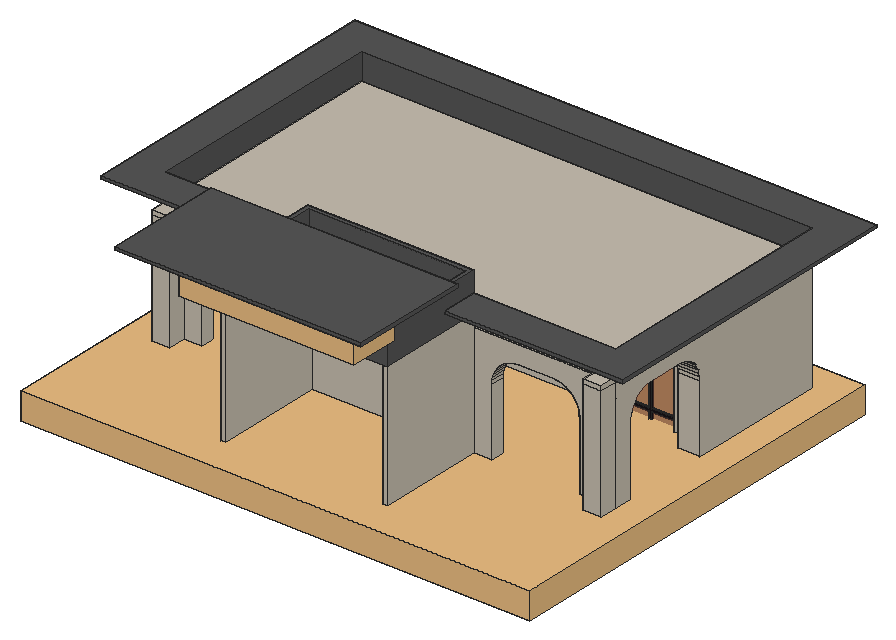
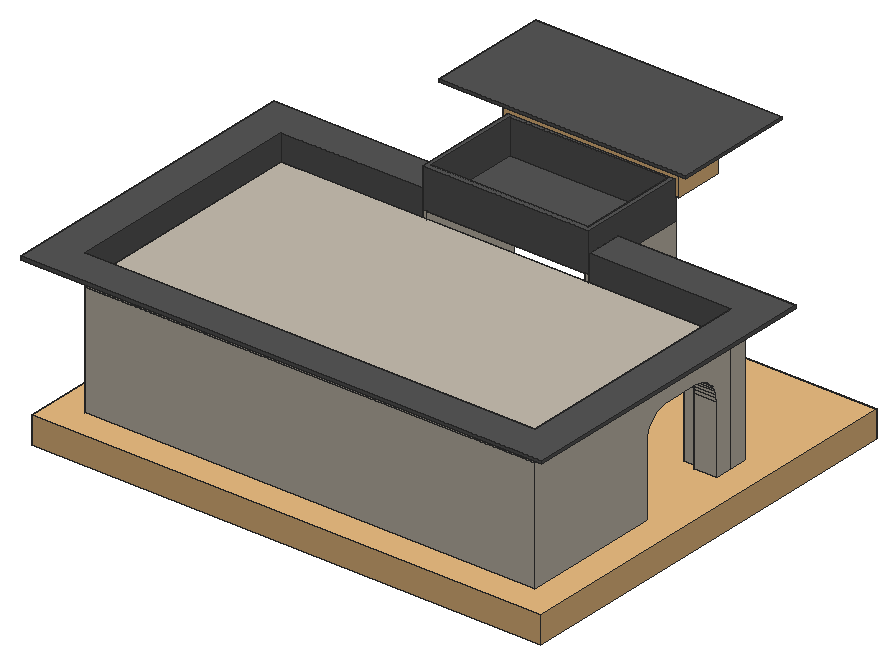
# SketchUp Ruby script. Lengths in inches.
U = 1.inch
M = Sketchup.active_model
def pt(a) = Geom::Point3d.new(a.map { |v| v * U })
def face(e, loops, mat)
  f = e.add_face(loops[0].map { |a| pt(a) })
  loops[1..].each { |l| e.add_face(l.map { |a| pt(a) }).erase! }
  f.material = f.back_material = mat if mat
  f
end
# faces: each face lists its corners as indices into pts; further lists are holes
def faces(e, pts, list, mat = nil) = list.each { |f| face(e, (f[0].is_a?(Array) ? f : [f]).map { |l| l.map { |i| pts[i] } }, mat) }
# xy, xz, yz: faces in a plane at the given z, y or x. An outline is a flat list of corners, or four numbers for a rectangle; further outlines are holes
def ring(l) = l.size == 4 ? [[l[0], l[1]], [l[2], l[1]], [l[2], l[3]], [l[0], l[3]]] : l.each_slice(2).to_a
def flat(e, list, mat, &to3) = list.each { |f| face(e, (f[0].is_a?(Array) ? f : [f]).map { |l| ring(l).map { |u, v| to3.(u, v) } }, mat) }
def xy(e, z, list, mat = nil) = flat(e, list, mat) { |x, y| [x, y, z] }
def xz(e, y, list, mat = nil) = flat(e, list, mat) { |x, z| [x, y, z] }
def yz(e, x, list, mat = nil) = flat(e, list, mat) { |y, z| [x, y, z] }
def lines(e, pts, list) = list.each { |a, b| e.add_line(pt(pts[a]), pt(pts[b])) }
# prism: a flat outline (further loops are holes) pulled along v
def prism(e, loops, v, mat = nil)
  f = face(e, loops, mat); d = Geom::Vector3d.new(v.map { |x| x * U })
  f.pushpull(f.normal.samedirection?(d) ? d.length : -d.length)
end
def box(e, o, s, mat = nil) = prism(e, [[o, [o[0] + s[0], o[1], o[2]], [o[0] + s[0], o[1] + s[1], o[2]], [o[0], o[1] + s[1], o[2]]]], [0, 0, s[2]], mat)
def at(x, y, z, deg = 0) = Geom::Transformation.translation(pt([x, y, z])) * Geom::Transformation.rotation(ORIGIN, Z_AXIS, deg.degrees)
def axes(o, x, y, z) = Geom::Transformation.new([*x, 0, *y, 0, *z, 0, *pt(o).to_a, 1])
def part(name) = M.definitions.add(name)
# library, detail: a bought-in or finely detailed component or shape, given as its bounding box
def library(name, o, s) = part(name).tap { |d| box(d.entities, o, s) }
def detail(e, o, s) = box(e.add_group.entities, o, s)
def put(e, d, t, mat = nil) = e.add_instance(d, t).tap { |i| i.material = mat if mat }
def group(e, t, mat = nil) = e.add_group.tap { |g| g.transformation = t; g.material = mat if mat }.entities
root = M.entities
M.materials.add("[0034_Wheat]").color = [198, 190, 175]
M.materials.add("[Carrera Marble]").color = [207, 207, 207]
M.materials.add("[Color M06]").color = [86, 86, 86]
M.materials.add("[Color M07]").color = [25, 20, 24]
M.materials.add("[Translucent Glass Dark Green]").color = [114, 59, 48]
M.materials["[Translucent Glass Dark Green]"].alpha = 0.5
c1 = library("Group\#14",[0,0,0],[679.6,559.6,36])
c2 = part("window")
xy(c2.entities,0,[[0,0,117,2]])
xy(c2.entities,3,[[3,0,38.5,2],[38.5,0,41.5,2],[41.5,0,75.5,2],[75.5,0,78.5,2],[78.5,0,114,2]])
xy(c2.entities,33,[[3,0,38.5,2],[41.5,0,75.5,2],[78.5,0,114,2]])
xy(c2.entities,36,[[3,0,38.5,2],[41.5,0,75.5,2],[78.5,0,114,2]])
xy(c2.entities,96,[[3,0,38.5,2],[41.5,0,75.5,2],[78.5,0,114,2]])
xy(c2.entities,99,[[3,0,38.5,2],[41.5,0,75.5,2],[78.5,0,114,2]])
xy(c2.entities,129,[[3,0,38.5,2],[41.5,0,75.5,2],[78.5,0,114,2]])
xy(c2.entities,132,[[0,0,117,2]])
xz(c2.entities,0,[[[0,0,117,132],[3,3,3,33,38.5,33,38.5,3,41.5,3,41.5,33,75.5,33,75.5,3,78.5,3,78.5,33,114,33,114,3],[3,36,38.5,96],[78.5,36,114,96],[41.5,36,75.5,96],[78.5,99,114,129],[3,99,38.5,129],[41.5,99,75.5,129]]])
xz(c2.entities,2,[[[0,0,117,132],[3,3,114,3,114,33,78.5,33,78.5,3,75.5,3,75.5,33,41.5,33,41.5,3,38.5,3,38.5,33,3,33],[3,36,38.5,96],[78.5,36,114,96],[41.5,36,75.5,96],[78.5,99,114,129],[3,99,38.5,129],[41.5,99,75.5,129]]])
xz(c2.entities,2,[[3,3,38.5,33],[41.5,3,75.5,33],[78.5,3,114,33],[3,36,38.5,96],[41.5,36,75.5,96],
  [78.5,36,114,96],[3,99,38.5,129],[41.5,99,75.5,129],[78.5,99,114,129]],"[Translucent Glass Dark Green]")
yz(c2.entities,0,[[0,0,2,132]])
yz(c2.entities,3,[[0,3,2,33],[0,36,2,96],[0,99,2,129]])
yz(c2.entities,38.5,[[0,3,2,33],[0,36,2,96],[0,99,2,129]])
yz(c2.entities,41.5,[[0,3,2,33],[0,36,2,96],[0,99,2,129]])
yz(c2.entities,75.5,[[0,3,2,33],[0,36,2,96],[0,99,2,129]])
yz(c2.entities,78.5,[[0,3,2,33],[0,36,2,96],[0,99,2,129]])
yz(c2.entities,114,[[0,3,2,33],[0,36,2,96],[0,99,2,129]])
yz(c2.entities,117,[[0,0,2,132]])
c3 = library("Group\#7",[-6.25,-50.07,0],[234.5,65.25,9.74])
p = [[237,110.43,204],[237,110.43,210]]
lines(root,p,[[0,1]])
g1 = group(root,at(48,101.43,204),"[0034_Wheat]")
xy(g1,0,[[0,0,0,480,600,480,600,0,411,0,411,153,189,153,189,0],[189,9,195,153],[405,9,411,153]])
xy(g1,6,[[0,0,189,0,189,153,411,153,411,0,600,0,600,480,0,480]],"[Carrera Marble]")
xy(g1,201,[[189,9,195,153],[405,9,411,153]])
xz(g1,0,[[0,0,189,6],[411,0,600,6]])
xz(g1,9,[[189,0,195,201],[405,0,411,201]])
xz(g1,153,[[189,0,195,6],[195,0,405,6],[405,0,411,6],[189,6,195,201],[405,6,411,201]])
xz(g1,480,[[0,0,600,6]])
yz(g1,0,[[0,0,480,6]])
yz(g1,189,[[0,0,9,6],[9,0,153,6],[9,6,153,201]])
yz(g1,195,[[9,0,153,201]])
yz(g1,405,[[9,0,153,201]])
yz(g1,411,[[0,0,9,6],[9,0,153,6],[9,6,153,201]])
yz(g1,600,[[0,0,480,6]])
put(root,c1,at(8.2,61.63,204),"[0034_Wheat]")
put(root,c2,axes([475.77,425.43,210],[1.06179,0,0],[0,1,0],[0,0,1.18182]),"[Color M07]")
put(root,c2,axes([96,425.43,210],[1.06179,0,0],[0,1,0],[0,0,1.18182]),"[Color M07]")
g2 = group(root,at(48,254.43,210),"[0034_Wheat]")
xy(g2,0,[[0,-24,24,0],[576,-24,600,0],[0,0,0,24,30,24,30,18,48,18,48,0],[165,0,435,18],[552,0,552,18,570,18,570,24,600,24,600,0],
  [0,141,0,327,600,327,600,141,570,141,570,297,30,297,30,171,54,171,54,165,30,165,30,141],[171,165,429,171],[546,165,570,171]])
xy(g2,156,[[84,0,129,18],[471,0,516,18],[0,60,30,105],[570,60,600,105],[90,165,135,171],
  [465,165,510,171]])
xy(g2,180,[[0,-24,24,0],[576,-24,600,0],[[0,0,600,327],[30,18,570,165],[30,171,570,297]]])
xy(g2,186,[[0,-24,24,0],[576,-24,600,0]])
xz(g2,-24,[[0,0,24,180],[576,0,600,180],[0,180,24,186],[576,180,600,186]])
xz(g2,0,[[0,0,24,180],[24,0,48,0,48,120,48.31,124.7,49.23,129.32,50.74,133.78,52.82,138,55.4375,141.92,58.54,145.46,62.08,148.5625,66,151.18,70.22,153.26,74.68,154.77,79.3,155.69,84,156,129,156,133.7,155.69,138.32,154.77,142.78,153.26,147,151.18,150.92,148.5625,154.46,145.46,157.5625,141.92,160.18,138,162.26,133.78,163.77,129.32,164.69,124.7,165,120,165,0,189,0,189,180,24,180],[189,0,411,180],[411,0,435,0,435,120,435.31,124.7,436.23,129.32,437.74,133.78,439.82,138,442.4375,141.92,445.54,145.46,449.08,148.5625,453,151.18,457.22,153.26,461.68,154.77,466.3,155.69,471,156,516,156,520.7,155.69,525.32,154.77,529.78,153.26,534,151.18,537.92,148.5625,541.46,145.46,544.5625,141.92,547.18,138,549.26,133.78,550.77,129.32,551.69,124.7,552,120,552,0,576,0,576,180,411,180],[576,0,600,180],
  [0,180,24,186],[576,180,600,186]])
xz(g2,18,[[30,0,30,180,570,180,570,0,552,0,552,120,551.69,124.7,550.77,129.32,549.26,133.78,547.18,138,544.5625,141.92,541.46,145.46,537.92,148.5625,534,151.18,529.78,153.26,525.32,154.77,520.7,155.69,516,156,471,156,466.3,155.69,461.68,154.77,457.22,153.26,453,151.18,449.08,148.5625,445.54,145.46,442.4375,141.92,439.82,138,437.74,133.78,436.23,129.32,435.31,124.7,435,120,435,0,165,0,165,120,164.69,124.7,163.77,129.32,162.26,133.78,160.18,138,157.5625,141.92,154.46,145.46,150.92,148.5625,147,151.18,142.78,153.26,138.32,154.77,133.7,155.69,129,156,84,156,79.3,155.69,74.68,154.77,70.22,153.26,66,151.18,62.08,148.5625,58.54,145.46,55.4375,141.92,52.82,138,50.74,133.78,49.23,129.32,48.31,124.7,48,120,48,0]])
xz(g2,24,[[0,0,30,120],[570,0,600,120]])
xz(g2,141,[[0,0,30,120],[570,0,600,120]])
xz(g2,165,[[30,0,54,0,54,120,54.31,124.7,55.23,129.32,56.74,133.78,58.82,138,61.4375,141.92,64.54,145.46,68.08,148.5625,72,151.18,76.22,153.26,80.68,154.77,85.3,155.69,90,156,135,156,139.7,155.69,144.32,154.77,148.78,153.26,153,151.18,156.92,148.5625,160.46,145.46,163.5625,141.92,166.18,138,168.26,133.78,169.77,129.32,170.69,124.7,171,120,171,0,429,0,429,120,429.31,124.7,430.23,129.32,431.74,133.78,433.82,138,436.4375,141.92,439.54,145.46,443.08,148.5625,447,151.18,451.22,153.26,455.68,154.77,460.3,155.69,465,156,510,156,514.7,155.69,519.32,154.77,523.78,153.26,528,151.18,531.92,148.5625,535.46,145.46,538.5625,141.92,541.18,138,543.26,133.78,544.77,129.32,545.69,124.7,546,120,546,0,570,0,570,180,30,180]])
xz(g2,171,[[30,0,30,180,570,180,570,0,546,0,546,120,545.69,124.7,544.77,129.32,543.26,133.78,541.18,138,538.5625,141.92,535.46,145.46,531.92,148.5625,528,151.18,523.78,153.26,519.32,154.77,514.7,155.69,510,156,465,156,460.3,155.69,455.68,154.77,451.22,153.26,447,151.18,443.08,148.5625,439.54,145.46,436.4375,141.92,433.82,138,431.74,133.78,430.23,129.32,429.31,124.7,429,120,429,0,171,0,171,120,170.69,124.7,169.77,129.32,168.26,133.78,166.18,138,163.5625,141.92,160.46,145.46,156.92,148.5625,153,151.18,148.78,153.26,144.32,154.77,139.7,155.69,135,156,90,156,85.3,155.69,80.68,154.77,76.22,153.26,72,151.18,68.08,148.5625,64.54,145.46,61.4375,141.92,58.82,138,56.74,133.78,55.23,129.32,54.31,124.7,54,120,54,0]])
xz(g2,297,[[30,0,570,180]])
xz(g2,327,[[0,0,600,180]])
yz(g2,0,[[-24,0,0,180],[0,0,0,180,327,180,327,0,141,0,141,120,140.69,124.7,139.77,129.32,138.26,133.78,136.18,138,133.5625,141.92,130.46,145.46,126.92,148.5625,123,151.18,118.78,153.26,114.32,154.77,109.7,155.69,105,156,60,156,55.3,155.69,50.68,154.77,46.22,153.26,42,151.18,38.08,148.5625,34.54,145.46,31.4375,141.92,28.82,138,26.74,133.78,25.23,129.32,24.31,124.7,24,120,24,0],[-24,180,0,186]])
yz(g2,24,[[-24,0,0,180],[-24,180,0,186]])
yz(g2,30,[[18,0,24,0,24,120,24.31,124.7,25.23,129.32,26.74,133.78,28.82,138,31.4375,141.92,34.54,145.46,38.08,148.5625,42,151.18,46.22,153.26,50.68,154.77,55.3,155.69,60,156,105,156,109.7,155.69,114.32,154.77,118.78,153.26,123,151.18,126.92,148.5625,130.46,145.46,133.5625,141.92,136.18,138,138.26,133.78,139.77,129.32,140.69,124.7,141,120,141,0,165,0,165,180,18,180],[171,0,297,180]])
yz(g2,48,[[0,0,18,120]])
yz(g2,54,[[165,0,171,120]])
yz(g2,165,[[0,0,18,120]])
yz(g2,171,[[165,0,171,120]])
yz(g2,429,[[165,0,171,120]])
yz(g2,435,[[0,0,18,120]])
yz(g2,546,[[165,0,171,120]])
yz(g2,552,[[0,0,18,120]])
yz(g2,570,[[18,0,18,180,165,180,165,0,141,0,141,120,140.69,124.7,139.77,129.32,138.26,133.78,136.18,138,133.5625,141.92,130.46,145.46,126.92,148.5625,123,151.18,118.78,153.26,114.32,154.77,109.7,155.69,105,156,60,156,55.3,155.69,50.68,154.77,46.22,153.26,42,151.18,38.08,148.5625,34.54,145.46,31.4375,141.92,28.82,138,26.74,133.78,25.23,129.32,24.31,124.7,24,120,24,0],[165,0,171,180],[171,0,297,180]])
yz(g2,576,[[-24,0,0,180],[-24,180,0,186]])
yz(g2,600,[[-24,0,0,180],[0,0,24,0,24,120,24.31,124.7,25.23,129.32,26.74,133.78,28.82,138,31.4375,141.92,34.54,145.46,38.08,148.5625,42,151.18,46.22,153.26,50.68,154.77,55.3,155.69,60,156,105,156,109.7,155.69,114.32,154.77,118.78,153.26,123,151.18,126.92,148.5625,130.46,145.46,133.5625,141.92,136.18,138,138.26,133.78,139.77,129.32,140.69,124.7,141,120,141,0,327,0,327,180,0,180],[-24,180,0,186]])
p = [[48.31,0,124.7],[48,0,120],[48,18,120],[48.31,18,124.7],[165,0,120],[164.69,0,124.7],
  [164.69,18,124.7],[165,18,120],[435.31,0,124.7],[435,0,120],[435,18,120],[435.31,18,124.7],
  [552,0,120],[551.69,0,124.7],[551.69,18,124.7],[552,18,120],[0,24,120],[0,24.31,124.7],
  [30,24.31,124.7],[30,24,120],[600,24.31,124.7],[600,24,120],[570,24,120],[570,24.31,124.7],
  [0,140.69,124.7],[0,141,120],[30,141,120],[30,140.69,124.7],[600,141,120],[600,140.69,124.7],
  [570,140.69,124.7],[570,141,120],[54.31,165,124.7],[54,165,120],[54,171,120],[54.31,171,124.7],
  [171,165,120],[170.69,165,124.7],[170.69,171,124.7],[171,171,120],[429.31,165,124.7],[429,165,120],
  [429,171,120],[429.31,171,124.7],[546,165,120],[545.69,165,124.7],[545.69,171,124.7],[546,171,120],
  [49.23,0,129.32],[49.23,18,129.32],[163.77,0,129.32],[163.77,18,129.32],[436.23,0,129.32],[436.23,18,129.32],
  [550.77,0,129.32],[550.77,18,129.32],[0,25.23,129.32],[30,25.23,129.32],[600,25.23,129.32],[570,25.23,129.32],
  [0,139.77,129.32],[30,139.77,129.32],[600,139.77,129.32],[570,139.77,129.32],[55.23,165,129.32],[55.23,171,129.32],
  [169.77,165,129.32],[169.77,171,129.32],[430.23,165,129.32],[430.23,171,129.32],[544.77,165,129.32],[544.77,171,129.32],
  [50.74,0,133.78],[50.74,18,133.78],[162.26,0,133.78],[162.26,18,133.78],[437.74,0,133.78],[437.74,18,133.78],
  [549.26,0,133.78],[549.26,18,133.78],[0,26.74,133.78],[30,26.74,133.78],[600,26.74,133.78],[570,26.74,133.78],
  [0,138.26,133.78],[30,138.26,133.78],[600,138.26,133.78],[570,138.26,133.78],[56.74,165,133.78],[56.74,171,133.78],
  [168.26,165,133.78],[168.26,171,133.78],[431.74,165,133.78],[431.74,171,133.78],[543.26,165,133.78],[543.26,171,133.78],
  [52.82,0,138],[52.82,18,138],[160.18,0,138],[160.18,18,138],[439.82,0,138],[439.82,18,138],
  [547.18,0,138],[547.18,18,138],[0,28.82,138],[30,28.82,138],[600,28.82,138],[570,28.82,138],
  [0,136.18,138],[30,136.18,138],[600,136.18,138],[570,136.18,138],[58.82,165,138],[58.82,171,138],
  [166.18,165,138],[166.18,171,138],[433.82,165,138],[433.82,171,138],[541.18,165,138],[541.18,171,138],
  [55.4375,0,141.92],[55.4375,18,141.92],[157.5625,0,141.92],[157.5625,18,141.92],[442.4375,0,141.92],[442.4375,18,141.92],
  [544.5625,0,141.92],[544.5625,18,141.92],[0,31.4375,141.92],[30,31.4375,141.92],[600,31.4375,141.92],[570,31.4375,141.92],
  [0,133.5625,141.92],[30,133.5625,141.92],[600,133.5625,141.92],[570,133.5625,141.92],[61.4375,165,141.92],[61.4375,171,141.92],
  [163.5625,165,141.92],[163.5625,171,141.92],[436.4375,165,141.92],[436.4375,171,141.92],[538.5625,165,141.92],[538.5625,171,141.92],
  [58.54,0,145.46],[58.54,18,145.46],[154.46,0,145.46],[154.46,18,145.46],[445.54,0,145.46],[445.54,18,145.46],
  [541.46,0,145.46],[541.46,18,145.46],[0,34.54,145.46],[30,34.54,145.46],[600,34.54,145.46],[570,34.54,145.46],
  [0,130.46,145.46],[30,130.46,145.46],[600,130.46,145.46],[570,130.46,145.46],[64.54,165,145.46],[64.54,171,145.46],
  [160.46,165,145.46],[160.46,171,145.46],[439.54,165,145.46],[439.54,171,145.46],[535.46,165,145.46],[535.46,171,145.46],
  [62.08,0,148.5625],[62.08,18,148.5625],[150.92,0,148.5625],[150.92,18,148.5625],[449.08,0,148.5625],[449.08,18,148.5625],
  [537.92,0,148.5625],[537.92,18,148.5625],[0,38.08,148.5625],[30,38.08,148.5625],[600,38.08,148.5625],[570,38.08,148.5625],
  [0,126.92,148.5625],[30,126.92,148.5625],[600,126.92,148.5625],[570,126.92,148.5625],[68.08,165,148.5625],[68.08,171,148.5625],
  [156.92,165,148.5625],[156.92,171,148.5625],[443.08,165,148.5625],[443.08,171,148.5625],[531.92,165,148.5625],[531.92,171,148.5625],
  [66,0,151.18],[66,18,151.18],[147,0,151.18],[147,18,151.18],[453,0,151.18],[453,18,151.18],
  [534,0,151.18],[534,18,151.18],[0,42,151.18],[30,42,151.18],[600,42,151.18],[570,42,151.18],
  [0,123,151.18],[30,123,151.18],[600,123,151.18],[570,123,151.18],[72,165,151.18],[72,171,151.18],
  [153,165,151.18],[153,171,151.18],[447,165,151.18],[447,171,151.18],[528,165,151.18],[528,171,151.18],
  [70.22,0,153.26],[70.22,18,153.26],[142.78,0,153.26],[142.78,18,153.26],[457.22,0,153.26],[457.22,18,153.26],
  [529.78,0,153.26],[529.78,18,153.26],[0,46.22,153.26],[30,46.22,153.26],[600,46.22,153.26],[570,46.22,153.26],
  [0,118.78,153.26],[30,118.78,153.26],[600,118.78,153.26],[570,118.78,153.26],[76.22,165,153.26],[76.22,171,153.26],
  [148.78,165,153.26],[148.78,171,153.26],[451.22,165,153.26],[451.22,171,153.26],[523.78,165,153.26],[523.78,171,153.26],
  [74.68,0,154.77],[74.68,18,154.77],[138.32,0,154.77],[138.32,18,154.77],[461.68,0,154.77],[461.68,18,154.77],
  [525.32,0,154.77],[525.32,18,154.77],[0,50.68,154.77],[30,50.68,154.77],[600,50.68,154.77],[570,50.68,154.77],
  [0,114.32,154.77],[30,114.32,154.77],[600,114.32,154.77],[570,114.32,154.77],[80.68,165,154.77],[80.68,171,154.77],
  [144.32,165,154.77],[144.32,171,154.77],[455.68,165,154.77],[455.68,171,154.77],[519.32,165,154.77],[519.32,171,154.77],
  [79.3,0,155.69],[79.3,18,155.69],[133.7,0,155.69],[133.7,18,155.69],[466.3,0,155.69],[466.3,18,155.69],
  [520.7,0,155.69],[520.7,18,155.69],[0,55.3,155.69],[30,55.3,155.69],[600,55.3,155.69],[570,55.3,155.69],
  [0,109.7,155.69],[30,109.7,155.69],[600,109.7,155.69],[570,109.7,155.69],[85.3,165,155.69],[85.3,171,155.69],
  [139.7,165,155.69],[139.7,171,155.69],[460.3,165,155.69],[460.3,171,155.69],[514.7,165,155.69],[514.7,171,155.69],
  [84,0,156],[84,18,156],[129,0,156],[129,18,156],[471,0,156],[471,18,156],
  [516,0,156],[516,18,156],[0,60,156],[30,60,156],[600,60,156],[570,60,156],
  [0,105,156],[30,105,156],[600,105,156],[570,105,156],[90,165,156],[90,171,156],
  [135,165,156],[135,171,156],[465,165,156],[465,171,156],[510,165,156],[510,171,156]]
faces(g2,p,[[0,1,2,3],[4,5,6,7],[8,9,10,11],[12,13,14,15],[16,17,18,19],[20,21,22,23],[24,25,26,27],[28,29,30,31],
  [32,33,34,35],[36,37,38,39],[40,41,42,43],[44,45,46,47],[48,0,3,49],[5,50,51,6],[52,8,11,53],[13,54,55,14],
  [17,56,57,18],[58,20,23,59],[60,24,27,61],[29,62,63,30],[64,32,35,65],[37,66,67,38],[68,40,43,69],[45,70,71,46],
  [72,48,49,73],[50,74,75,51],[76,52,53,77],[54,78,79,55],[56,80,81,57],[82,58,59,83],[84,60,61,85],[62,86,87,63],
  [88,64,65,89],[66,90,91,67],[92,68,69,93],[70,94,95,71],[96,72,73,97],[74,98,99,75],[100,76,77,101],[78,102,103,79],
  [80,104,105,81],[106,82,83,107],[108,84,85,109],[86,110,111,87],[112,88,89,113],[90,114,115,91],[116,92,93,117],[94,118,119,95],
  [120,96,97,121],[98,122,123,99],[124,100,101,125],[102,126,127,103],[104,128,129,105],[130,106,107,131],[132,108,109,133],[110,134,135,111],
  [136,112,113,137],[114,138,139,115],[140,116,117,141],[118,142,143,119],[144,120,121,145],[122,146,147,123],[148,124,125,149],[126,150,151,127],
  [128,152,153,129],[154,130,131,155],[156,132,133,157],[134,158,159,135],[160,136,137,161],[138,162,163,139],[164,140,141,165],[142,166,167,143],
  [168,144,145,169],[146,170,171,147],[172,148,149,173],[150,174,175,151],[152,176,177,153],[178,154,155,179],[180,156,157,181],[158,182,183,159],
  [184,160,161,185],[162,186,187,163],[188,164,165,189],[166,190,191,167],[192,168,169,193],[170,194,195,171],[196,172,173,197],[174,198,199,175],
  [176,200,201,177],[202,178,179,203],[204,180,181,205],[182,206,207,183],[208,184,185,209],[186,210,211,187],[212,188,189,213],[190,214,215,191],
  [216,192,193,217],[194,218,219,195],[220,196,197,221],[198,222,223,199],[200,224,225,201],[226,202,203,227],[228,204,205,229],[206,230,231,207],
  [232,208,209,233],[210,234,235,211],[236,212,213,237],[214,238,239,215],[240,216,217,241],[218,242,243,219],[244,220,221,245],[222,246,247,223],
  [224,248,249,225],[250,226,227,251],[252,228,229,253],[230,254,255,231],[256,232,233,257],[234,258,259,235],[260,236,237,261],[238,262,263,239],
  [264,240,241,265],[242,266,267,243],[268,244,245,269],[246,270,271,247],[248,272,273,249],[274,250,251,275],[276,252,253,277],[254,278,279,255],
  [280,256,257,281],[258,282,283,259],[284,260,261,285],[262,286,287,263],[288,264,265,289],[266,290,291,267],[292,268,269,293],[270,294,295,271],
  [272,296,297,273],[298,274,275,299],[300,276,277,301],[278,302,303,279],[304,280,281,305],[282,306,307,283],[308,284,285,309],[286,310,311,287]])
g3 = group(root,at(48,254.43,390),"[0034_Wheat]")
box(g3,[0,0,0],[600,327,6])
g4 = group(root,at(48,254.43,396),"[Color M06]")
xy(g4,34.625,[[-48,-48,189,-48,189,0,0,0,0,327,600,327,600,0,411,0,411,-48,648,-48,648,375,-48,375]])
xz(g4,-48,[[-48,30.625,189,34.625],[411,30.625,648,34.625]])
xz(g4,0,[[0,0,189,34.625],[411,0,600,34.625]])
xz(g4,327,[[0,0,600,34.625]])
xz(g4,375,[[-48,30.625,648,34.625]])
yz(g4,-48,[[-48,30.625,375,34.625]])
yz(g4,0,[[0,0,327,34.625]])
yz(g4,189,[[0,0,0,34.625,-48,34.625,-48,30.625]])
yz(g4,411,[[0,0,-48,30.625,-48,34.625,0,34.625]])
yz(g4,600,[[0,0,327,34.625]])
yz(g4,648,[[-48,30.625,375,34.625]])
p = [[-48,375,30.625],[0,327,0],[0,0,0],[-48,-48,30.625],[189,0,0],[189,-48,30.625],
  [600,0,0],[648,-48,30.625],[411,-48,30.625],[411,0,0],[600,327,0],[648,375,30.625]]
faces(g4,p,[[0,1,2,3],[3,2,4,5],[6,7,8,9],[10,11,7,6],[11,10,1,0]])
g5 = group(root,at(237,110.43,405),"[Color M06]")
xy(g5,0,[[0,0,222,144]])
xy(g5,6,[[6,6,216,138]])
xy(g5,52.6875,[[[0,0,222,144],[6,6,216,138]]])
xz(g5,0,[[0,0,222,52.6875]])
xz(g5,6,[[6,6,216,52.6875]])
xz(g5,138,[[6,6,216,52.6875]])
xz(g5,144,[[0,0,222,52.6875]])
yz(g5,0,[[0,0,144,52.6875]])
yz(g5,6,[[6,6,138,52.6875]])
yz(g5,216,[[6,6,138,52.6875]])
yz(g5,222,[[0,0,144,52.6875]])
put(root,c3,axes([237,97.25,437.26],[1,0,0],[0,1,0],[0,0,3]),"[0034_Wheat]")
g6 = group(root,at(183.57,0,466.49),"[Color M06]")
xy(g6,0,[[48,48,280.86,112.43]])
xy(g6,34.625,[[0,0,328.86,160.43]])
xz(g6,0,[[0,30.625,328.86,34.625]])
xz(g6,160.43,[[0,30.625,328.86,34.625]])
yz(g6,0,[[0,30.625,160.43,34.625]])
yz(g6,328.86,[[0,30.625,160.43,34.625]])
p = [[48,48,0],[0,0,30.625],[0,160.43,30.625],[48,112.43,0],[280.86,48,0],[328.86,0,30.625],
  [280.86,112.43,0],[328.86,160.43,30.625]]
faces(g6,p,[[0,1,2,3],[4,5,1,0],[6,7,5,4],[3,2,7,6]])
